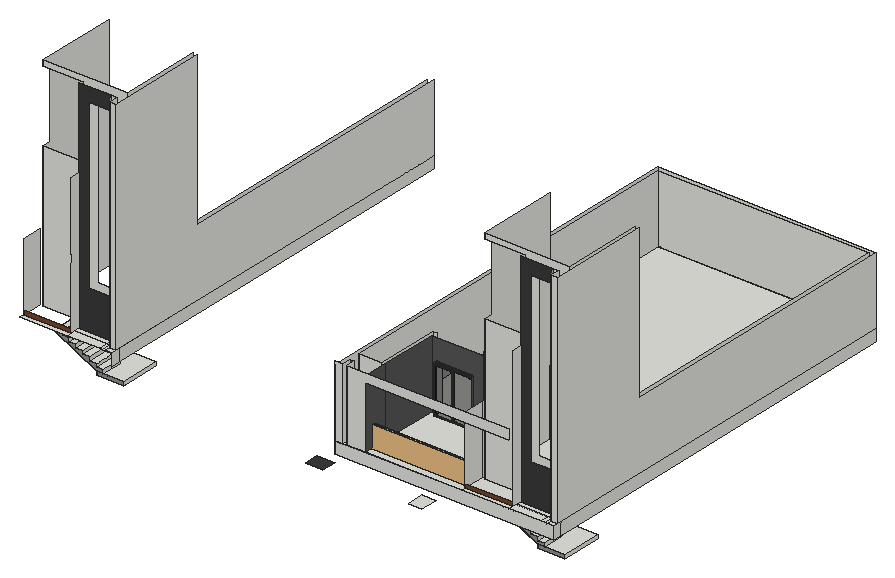
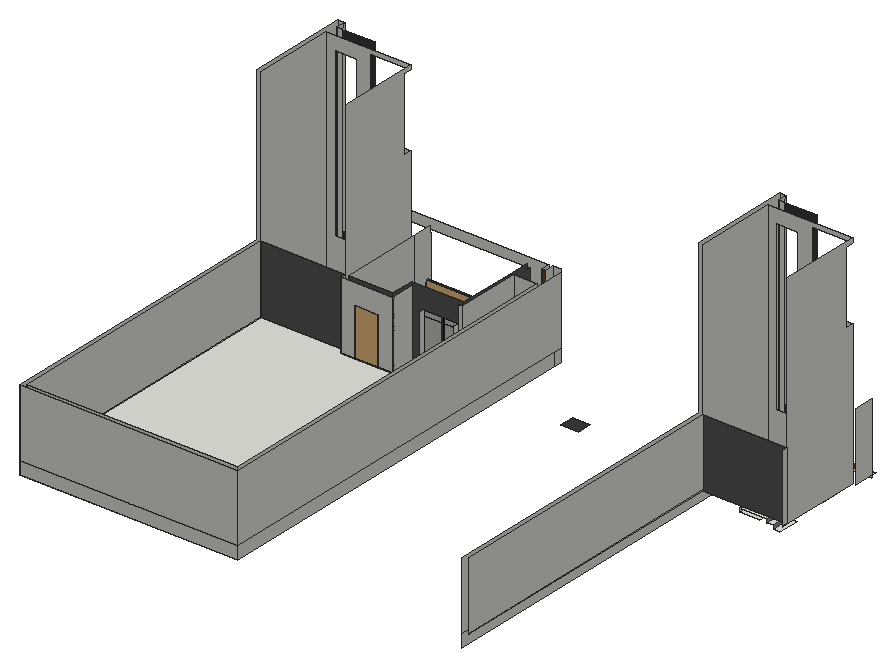
# SketchUp Ruby script. Lengths in inches.
U = 1.inch
M = Sketchup.active_model
def pt(a) = Geom::Point3d.new(a.map { |v| v * U })
def face(e, loops, mat)
  f = e.add_face(loops[0].map { |a| pt(a) })
  loops[1..].each { |l| e.add_face(l.map { |a| pt(a) }).erase! }
  f.material = f.back_material = mat if mat
  f
end
# faces: each face lists its corners as indices into pts; further lists are holes
def faces(e, pts, list, mat = nil) = list.each { |f| face(e, (f[0].is_a?(Array) ? f : [f]).map { |l| l.map { |i| pts[i] } }, mat) }
# xy, xz, yz: faces in a plane at the given z, y or x. An outline is a flat list of corners, or four numbers for a rectangle; further outlines are holes
def ring(l) = l.size == 4 ? [[l[0], l[1]], [l[2], l[1]], [l[2], l[3]], [l[0], l[3]]] : l.each_slice(2).to_a
def flat(e, list, mat, &to3) = list.each { |f| face(e, (f[0].is_a?(Array) ? f : [f]).map { |l| ring(l).map { |u, v| to3.(u, v) } }, mat) }
def xy(e, z, list, mat = nil) = flat(e, list, mat) { |x, y| [x, y, z] }
def xz(e, y, list, mat = nil) = flat(e, list, mat) { |x, z| [x, y, z] }
def yz(e, x, list, mat = nil) = flat(e, list, mat) { |y, z| [x, y, z] }
def lines(e, pts, list) = list.each { |a, b| e.add_line(pt(pts[a]), pt(pts[b])) }
# prism: a flat outline (further loops are holes) pulled along v
def prism(e, loops, v, mat = nil)
  f = face(e, loops, mat); d = Geom::Vector3d.new(v.map { |x| x * U })
  f.pushpull(f.normal.samedirection?(d) ? d.length : -d.length)
end
def box(e, o, s, mat = nil) = prism(e, [[o, [o[0] + s[0], o[1], o[2]], [o[0] + s[0], o[1] + s[1], o[2]], [o[0], o[1] + s[1], o[2]]]], [0, 0, s[2]], mat)
def at(x, y, z, deg = 0) = Geom::Transformation.translation(pt([x, y, z])) * Geom::Transformation.rotation(ORIGIN, Z_AXIS, deg.degrees)
def axes(o, x, y, z) = Geom::Transformation.new([*x, 0, *y, 0, *z, 0, *pt(o).to_a, 1])
def part(name) = M.definitions.add(name)
# library, detail: a bought-in or finely detailed component or shape, given as its bounding box
def library(name, o, s) = part(name).tap { |d| box(d.entities, o, s) }
def detail(e, o, s) = box(e.add_group.entities, o, s)
def put(e, d, t, mat = nil) = e.add_instance(d, t).tap { |i| i.material = mat if mat }
def group(e, t, mat = nil) = e.add_group.tap { |g| g.transformation = t; g.material = mat if mat }.entities
root = M.entities
M.materials.add("Glass_Tinted_Gray").color = [0, 0, 0]
M.materials["Glass_Tinted_Gray"].alpha = 0.125
M.materials.add("[0135_DarkGray]").color = [81, 81, 81]
M.materials.add("[Blacktop Old 02]").color = [143, 145, 145]
M.materials.add("[Color M06]").color = [86, 86, 86]
M.materials.add("[Color M07]").color = [58, 58, 58]
M.materials.add("[Mirror 02]").color = [229, 229, 229]
M.materials.add("[Terrazzo Light Blue]").color = [196, 214, 227]
M.materials.add("[Wood Floor Dark]").color = [153, 94, 42]
M.materials.add("[Wood Veneer 01]").color = [120, 70, 37]
c1 = part("PENTEK_RP Fineline 50S_Sliding_DoorCase_E1")
box(c1.entities,[0,0,0],[1.51,3.66,99.27],"[0135_DarkGray]")
c2 = part("PENTEK_RP Fineline 50S_SlidingDooe_Case_E2")
box(c2.entities,[0,0,0],[96.25,3.66,1.51],"[0135_DarkGray]")
c3 = part("pentek_RP Fineline 50S_SlidingDoor_Case")
put(c3.entities,c1,at(97.76,0,0))
put(c3.entities,c2,at(1.51,0,0))
put(c3.entities,c1,at(0,0,0))
put(c3.entities,c2,at(1.51,0,97.76))
c4 = part("PENTEK_RP Fineline 50S_SlidingDoor_GlazingBead_2")
box(c4.entities,[0,0,0],[0.56,0.59,94.39],"[0135_DarkGray]")
c5 = part("PENTEK_RP Fineline 50S_SlidingDoor_Glass")
box(c5.entities,[0,0,0],[46.58,0.16,94.39],"Glass_Tinted_Gray")
c6 = part("PENTEK_RP Fineline 50S_SlidingDoor_GlazingBead")
box(c6.entities,[0,0,0],[45.47,0.59,0.56],"[0135_DarkGray]")
c7 = part("PENTEK_RP Fineline 50S_SlidingDoor_Leaf_E1")
xy(c7.entities,0,[[0,0,0.93,1.97],[0.93,1.57,1.49,1.97]],"[0135_DarkGray]")
xy(c7.entities,96.25,[[0,0,0.93,0,0.93,1.57,1.49,1.57,1.49,1.97,0,1.97]],"[0135_DarkGray]")
xz(c7.entities,0,[[0,0,0.93,96.25]],"[0135_DarkGray]")
xz(c7.entities,1.57,[[0.93,0,1.49,95.32],[0.93,95.32,1.49,96.25]],"[0135_DarkGray]")
xz(c7.entities,1.97,[[0,0,1.49,96.25]],"[0135_DarkGray]")
yz(c7.entities,0,[[0,0,1.97,96.25]],"[0135_DarkGray]")
yz(c7.entities,0.93,[[0,0,1.57,0.93],[0,0.93,1.57,95.32],[0,95.32,1.57,96.25]],"[0135_DarkGray]")
yz(c7.entities,1.49,[[1.57,0,1.97,95.32],[1.57,95.32,1.97,96.25]],"[0135_DarkGray]")
c8 = part("PENTEK_RP Fineline 50S_SlidingDoor_Leaf_E2")
xy(c8.entities,0,[[0,0,0,1.57,0.56,1.57,0.56,1.97,46.02,1.97,46.02,1.57,46.58,1.57,46.58,0]],"[0135_DarkGray]")
xy(c8.entities,0.93,[[0,0,46.58,1.57]],"[0135_DarkGray]")
xy(c8.entities,1.49,[[0.56,1.57,46.02,1.97]],"[0135_DarkGray]")
xz(c8.entities,0,[[0,0,46.58,0.93]],"[0135_DarkGray]")
xz(c8.entities,1.57,[[0,0,0.56,0.93],[46.02,0,46.58,0.93],[0.56,0.93,46.02,1.49]],"[0135_DarkGray]")
xz(c8.entities,1.97,[[0.56,0,46.02,1.49]],"[0135_DarkGray]")
yz(c8.entities,0,[[0,0,1.57,0.93]],"[0135_DarkGray]")
yz(c8.entities,0.56,[[1.57,0,1.97,0.93],[1.57,0.93,1.97,1.49]],"[0135_DarkGray]")
yz(c8.entities,46.02,[[1.57,0,1.97,0.93],[1.57,0.93,1.97,1.49]],"[0135_DarkGray]")
yz(c8.entities,46.58,[[0,0,1.57,0.93]],"[0135_DarkGray]")
c9 = part("PENTEK_RP Fineline S_SlidingDoor_Leaf1")
put(c9.entities,c4,at(0.93,0,0.93))
put(c9.entities,c4,at(46.96,0,0.93))
put(c9.entities,c5,at(1.49,1.42,0.93))
put(c9.entities,c6,at(1.49,0,0.93))
put(c9.entities,c5,at(1.49,0.59,0.93),"[Terrazzo Light Blue]")
put(c9.entities,c7,at(0,0,0))
put(c9.entities,c7,axes([48.44,0,0],[-1,0,0],[0,1,0],[0,0,1]))
put(c9.entities,c8,axes([0.93,0,96.25],[1,0,0],[0,1,0],[0,0,-1]))
put(c9.entities,c8,at(0.93,0,0))
put(c9.entities,c6,at(1.49,0,94.77))
c10 = part("PENTEK_RP Fineline 50S_SlidingDoor_Leaf2")
put(c10.entities,c5,at(1.49,1.42,0.93))
put(c10.entities,c6,at(1.49,0,94.77))
put(c10.entities,c4,at(46.96,0,0.93))
put(c10.entities,c5,at(1.49,0.59,0.93),"[Mirror 02]")
put(c10.entities,c4,at(0.93,0,0.93))
put(c10.entities,c7,at(0,0,0))
put(c10.entities,c7,axes([48.44,0,0],[-1,0,0],[0,1,0],[0,0,1]))
put(c10.entities,c6,at(1.49,0,0.93))
put(c10.entities,c8,axes([0.93,0,96.25],[1,0,0],[0,1,0],[0,0,-1]))
put(c10.entities,c8,at(0.93,0,0))
c11 = part("PENTEK - Slimmest Steel Sliding Door / Window\#1")
put(c11.entities,c3,at(0,-1.88,-0.09))
put(c11.entities,c9,at(1.51,-2.27,1.42))
put(c11.entities,c10,at(49.32,-0.3,1.42))
c12 = library("Glass Railing",[0,0,0],[139.5,4.76,42])
c13 = library("door (1)",[38.93,25.48,0],[40,9.94,82.68])
xy(root,69.625,[[2545.07,297.1875,2568.82,327.09]])
xy(root,69.625,[[2363.46,297,2394.2,321.97]],"[Color M07]")
xy(root,71.875,[[1967.4,335.33,1979.4,371.33],[2747.78,335.33,2759.78,371.33]])
xy(root,77.875,[[1991.4,299.33,1991.4,335.33,2003.4,335.33,2003.4,371.33,2039.4,371.33,2039.4,299.33],[2771.78,299.33,2771.78,335.33,2783.78,335.33,2783.78,371.33,2819.78,371.33,2819.78,299.33],[1979.4,335.33,1991.4,371.33],[2759.78,335.33,2771.78,371.33]])
xy(root,83.875,[[1991.4,299.33,2003.4,335.33],[2003.4,299.33,2039.4,299.33,2039.4,371.33,1991.4,371.33,1991.4,335.33,2003.4,335.33],[2771.78,299.33,2783.78,335.33],[2783.78,299.33,2819.78,299.33,2819.78,371.33,2771.78,371.33,2771.78,335.33,2783.78,335.33]])
xy(root,89.875,[[1991.4,299.33,2003.4,335.33],[2771.78,299.33,2783.78,335.33]])
xy(root,94.0625,[[2488.8,431.33,2550.55,440.27]])
xy(root,95.875,[[1979.4,299.33,1991.4,335.33],[2759.78,299.33,2771.78,335.33]])
xy(root,101.875,[[1967.4,299.33,1979.4,335.33],[2747.78,299.33,2759.78,335.33]])
xy(root,107.875,[[1955.4,299.33,1967.4,335.33],[2735.78,299.33,2747.78,335.33]])
xy(root,113.875,[[1943.4,299.33,1955.4,335.33],[2723.78,299.33,2735.78,335.33]])
xy(root,119.875,[[1931.4,299.33,1943.4,335.33],[2711.78,299.33,2723.78,335.33]])
xy(root,125.875,[[2441.46,264.125,2827.34,279.8125],[1919.4,299.33,1931.4,335.33],[2699.78,299.33,2711.78,335.33],[[2627.78,371.33,2627.78,431.33,2441.46,431.33,2441.46,975.9375,2827.34,975.9375,2827.34,371.33],[2633.78,379.21,2822.07,379.21,2822.07,970.67,2446.73,970.67,2446.73,440.27,2633.78,440.27]]])
xy(root,125.875,[[[2441.46,279.8125,2441.46,431.33,2627.78,431.33,2627.78,371.33,2827.34,371.33,2827.34,279.8125],[2699.78,299.33,2711.78,335.33],[2446.73,334.62,2454.1,350.3]]],"[Wood Floor Dark]")
xy(root,147.1875,[[2448.71,308.24,2448.71,968.69,2820.09,968.69,2820.09,452.5625,2670.45,452.5625,2670.45,462.67,2579.54,462.67,2579.54,420.39,2538.36,421.04,2488.82,421.04,2488.82,308.24]])
xy(root,147.625,[[1884.4,264.125,1968.34,272.125],[1968.34,264.125,2025.4,279.8125],[2025.4,264.125,2031.45,279.8125],[2031.45,264.125,2035.66,264.125,2035.66,273.0625,2031.45,279.8125],[2035.66,264.125,2046.96,273.0625],
  [2441.46,264.125,2455.02,279.8125],[2455.02,264.125,2462.375,279.8125],[2462.375,264.125,2494.84,279.8125],[2494.84,264.125,2664.78,279.8125],[2664.78,264.125,2748.72,272.125],
  [2748.72,264.125,2805.78,279.8125],[2805.78,264.125,2811.82,279.8125],[2811.82,264.125,2816.04,264.125,2816.04,273.0625,2811.82,279.8125],[2816.04,264.125,2827.34,273.0625],[1884.4,272.125,1968.34,273.0625],
  [2664.78,272.125,2748.72,273.0625],[1884.4,273.0625,1968.34,279.8125],[2035.66,273.0625,2035.66,279.8125,2031.45,279.8125],[2035.66,273.0625,2046.96,279.8125],[2664.78,273.0625,2748.72,279.8125],
  [2816.04,273.0625,2816.04,279.8125,2811.82,279.8125],[2816.04,273.0625,2827.34,279.8125],[1968.34,279.8125,2025.4,289.5],[2025.4,279.8125,2031.45,279.8125,2025.4,289.5],[2031.45,279.8125,2025.4,289.5,2035.66,289.5,2035.66,279.8125],
  [2441.46,279.8125,2441.46,975.9375,2827.34,975.9375,2827.34,279.8125,2816.04,279.8125,2816.04,289.5,2748.72,289.5,2748.72,279.8125,2664.78,279.8125,2664.78,452.5625,2646.47,452.5625,2646.47,462.67,2670.45,462.67,2670.45,308.24,2820.09,308.24,2820.09,968.69,2448.71,968.69,2448.71,308.24,2488.82,308.24,2488.82,421.04,2503.97,421.04,2503.97,411.0625,2494.84,411.0625,2494.84,279.8125],[2494.84,279.8125,2664.78,308.24],[2748.72,279.8125,2805.78,289.5],[2805.78,279.8125,2811.82,279.8125,2805.78,289.5],[2811.82,279.8125,2805.78,289.5,2816.04,289.5,2816.04,279.8125],
  [2448.71,308.24,2448.71,968.69,2820.09,968.69,2820.09,308.24,2670.45,308.24,2670.45,462.67,2579.54,462.67,2579.54,420.39,2565.72,420.61,2538.36,421.04,2488.82,421.04,2488.82,308.24],[2494.84,308.24,2664.78,308.24,2664.78,452.5625,2646.47,452.5625,2646.47,462.67,2604.72,462.67,2604.72,452.5625,2586.59,452.5625,2586.59,411.0625,2565.72,411.0625,2565.72,420.61,2503.97,420.61,2503.97,411.0625,2494.84,411.0625],[2565.72,411.0625,2565.72,420.61,2579.54,420.39,2579.54,462.67,2604.72,462.67,2604.72,452.5625,2586.59,452.5625,2586.59,411.0625],[2503.97,420.61,2503.97,421.04,2538.36,421.04,2565.72,420.61]])
xz(root,264.125,[[2441.46,125.875,2827.34,147.625],[2441.46,147.625,2455.02,273.625],[2462.375,147.625,2494.84,147.625,2494.84,256.875,2748.72,256.875,2748.72,273.625,2462.375,273.625]])
xz(root,272.125,[[1884.4,147.625,1968.34,154.375],[2664.78,147.625,2748.72,154.375]],"[Wood Veneer 01]")
xz(root,273.0625,[[1884.4,143.05,1968.34,147.625],[2664.78,143.05,2748.72,147.625],[2035.66,147.625,2046.96,536.4375],[2816.04,147.625,2827.34,536.4375]])
xz(root,279.8125,[[2441.46,125.875,2827.34,147.625]])
xz(root,279.8125,[[2455.02,147.625,2462.375,273.625]],"[Wood Veneer 01]")
xz(root,289.5,[[2025.4,147.625,2035.66,536.4375],[2805.78,147.625,2816.04,536.4375]])
xz(root,289.5,[[1968.34,147.625,2025.4,147.625,2025.4,217.36,1986.53,217.36,1986.53,512.23,2025.4,512.23,2025.4,536.4375,1968.34,536.4375],[2748.72,147.625,2805.78,147.625,2805.78,217.36,2766.9,217.36,2766.9,512.23,2805.78,512.23,2805.78,536.4375,2748.72,536.4375]],"[Color M07]")
xz(root,299.33,[[1991.4,77.875,2039.4,83.875],[2771.78,77.875,2819.78,83.875],[1991.4,83.875,2003.4,83.875,2003.4,89.875,1991.4,89.875,1991.4,95.875,1979.4,95.875,1979.4,101.875,1967.4,101.875,1967.4,107.875,1955.4,107.875,1955.4,113.875,1943.4,113.875,1943.4,119.875,1931.4,119.875,1931.4,125.875,1919.4,125.875,1919.4,119.875],[2771.78,83.875,2783.78,83.875,2783.78,89.875,2771.78,89.875,2771.78,95.875,2759.78,95.875,2759.78,101.875,2747.78,101.875,2747.78,107.875,2735.78,107.875,2735.78,113.875,2723.78,113.875,2723.78,119.875,2711.78,119.875,2711.78,125.875,2699.78,125.875,2699.78,119.875]],"[Blacktop Old 02]")
xz(root,308.24,[[2448.71,147.1875,2488.82,147.625],[[1890.08,147.625,1890.08,400.68,1962.22,400.68,1962.22,528.11,1890.08,528.11,1890.08,536.4375,2039.72,536.4375,2039.72,147.625],[1986.53,217.36,2025.4,512.23]],[2448.71,147.625,2488.82,267.625],[[2670.45,147.625,2670.45,400.68,2742.59,400.68,2742.59,528.11,2670.45,528.11,2670.45,536.4375,2820.09,536.4375,2820.09,147.625],[2766.9,217.36,2805.78,512.23]]])
xz(root,335.33,[[1991.4,83.875,1919.4,119.875,1919.4,125.875,1931.4,125.875,1931.4,119.875,1943.4,119.875,1943.4,113.875,1955.4,113.875,1955.4,107.875,1967.4,107.875,1967.4,101.875,1979.4,101.875,1979.4,95.875,1991.4,95.875,1991.4,89.875,2003.4,89.875,2003.4,83.875],[2771.78,83.875,2699.78,119.875,2699.78,125.875,2711.78,125.875,2711.78,119.875,2723.78,119.875,2723.78,113.875,2735.78,113.875,2735.78,107.875,2747.78,107.875,2747.78,101.875,2759.78,101.875,2759.78,95.875,2771.78,95.875,2771.78,89.875,2783.78,89.875,2783.78,83.875]])
xz(root,411.0625,[[2494.84,147.625,2503.97,147.625,2503.97,230.5625,2565.72,230.5625,2565.72,147.625,2586.59,147.625,2586.59,267.625,2494.84,267.625]],"[Color M06]")
xz(root,421.04,[[2488.82,147.1875,2496.09,147.625],[2496.09,147.1875,2538.36,147.625],[2488.82,147.625,2496.09,267.625]])
xz(root,452.5625,[[1890.08,147.1875,2039.72,267.625],[2670.45,147.1875,2820.09,267.625],[2586.59,147.625,2604.72,147.625,2604.72,231.75,2646.47,231.75,2646.47,147.625,2664.78,147.625,2664.78,267.625,2586.59,267.625]],"[Color M06]")
xz(root,462.67,[[2579.54,147.1875,2670.45,147.625],[2579.54,147.625,2604.72,147.625,2604.72,231.75,2646.47,231.75,2646.47,147.625,2670.45,147.625,2670.45,267.625,2579.54,267.625]])
xz(root,968.69,[[2448.71,147.1875,2820.09,147.625],[2448.71,147.625,2820.09,267.625]])
xz(root,975.9375,[[2441.46,125.875,2827.34,147.625],[2441.46,147.625,2827.34,267.625]])
yz(root,1884.4,[[272.125,147.625,272.125,154.375,273.0625,154.375,273.0625,155.86,272.125,155.86,272.125,167.1875,273.0625,167.1875,273.0625,168.67,272.125,168.67,272.125,180,273.0625,180,273.0625,181.48,272.125,181.48,272.125,192.8125,273.0625,192.8125,273.0625,194.3,272.125,194.3,272.125,205.625,273.0625,205.625,273.0625,207.11,272.125,207.11,272.125,218.4375,273.0625,218.4375,273.0625,219.92,272.125,219.92,272.125,231.25,273.0625,231.25,273.0625,232.73,272.125,232.73,272.125,244.0625,273.0625,244.0625,273.0625,245.55,272.125,245.55,272.125,256.875,273.0625,256.875,273.0625,267.625,308.24,267.625,308.24,147.625]])
yz(root,1890.08,[[452.5625,147.1875,462.67,147.625],[308.24,147.625,452.5625,147.625,452.5625,536.4375,308.24,536.4375,308.24,528.11,323.81,528.11,323.81,400.68,308.24,400.68],[452.5625,147.625,462.67,267.625]])
yz(root,1919.4,[[299.33,119.875,335.33,125.875]])
yz(root,1931.4,[[299.33,119.875,335.33,125.875]])
yz(root,1943.4,[[299.33,113.875,335.33,119.875]])
yz(root,1955.4,[[299.33,107.875,335.33,113.875]])
yz(root,1967.4,[[299.33,101.875,335.33,107.875]])
yz(root,1968.34,[[272.125,147.625,289.5,147.625,289.5,393.625,271.6875,393.625,271.6875,273.625,273.0625,273.625,273.0625,256.875,272.125,256.875,272.125,245.55,273.0625,245.55,273.0625,244.0625,272.125,244.0625,272.125,232.73,273.0625,232.73,273.0625,231.25,272.125,231.25,272.125,219.92,273.0625,219.92,273.0625,218.4375,272.125,218.4375,272.125,207.11,273.0625,207.11,273.0625,205.625,272.125,205.625,272.125,194.3,273.0625,194.3,273.0625,192.8125,272.125,192.8125,272.125,181.48,273.0625,181.48,273.0625,180,272.125,180,272.125,168.67,273.0625,168.67,273.0625,167.1875,272.125,167.1875,272.125,155.86,273.0625,155.86,273.0625,154.375,272.125,154.375]])
yz(root,1979.4,[[299.33,95.875,335.33,101.875]])
yz(root,1979.4,[[335.33,71.875,371.33,77.875]],"[Blacktop Old 02]")
yz(root,1991.4,[[299.33,89.875,335.33,95.875]])
yz(root,1991.4,[[299.33,77.875,335.33,83.875],[335.33,77.875,371.33,83.875]],"[Blacktop Old 02]")
yz(root,2003.4,[[299.33,83.875,335.33,89.875]])
yz(root,2035.66,[[273.0625,147.625,289.5,536.4375]])
yz(root,2039.4,[[299.33,77.875,371.33,83.875]])
yz(root,2039.72,[[452.5625,147.1875,968.69,147.625],[308.24,147.625,452.5625,536.4375],[452.5625,147.625,968.69,267.625]])
yz(root,2046.96,[[264.125,125.875,279.8125,147.625],[279.8125,125.875,975.9375,147.625],[273.0625,147.625,975.9375,147.625,975.9375,267.625,452.5625,267.625,452.5625,536.4375,273.0625,536.4375]])
yz(root,2441.46,[[264.125,125.875,279.8125,147.625],[279.8125,125.875,975.9375,147.625],[264.125,147.625,975.9375,267.625]])
yz(root,2448.71,[[308.24,147.1875,968.69,147.625],[308.24,147.625,968.69,267.625]])
yz(root,2455.02,[[264.125,147.625,279.8125,273.625]])
yz(root,2462.375,[[264.125,147.625,279.8125,273.625]])
yz(root,2488.82,[[308.24,147.1875,421.04,147.625],[308.24,147.625,421.04,267.625]])
yz(root,2494.84,[[264.125,147.625,308.24,147.625,308.24,267.625,272.68,267.625,272.68,256.875,264.125,256.875],[308.24,147.625,411.0625,267.625]],"[Color M06]")
yz(root,2503.97,[[411.0625,147.625,420.61,230.5625]])
yz(root,2565.72,[[411.0625,147.625,420.61,230.5625]])
yz(root,2579.54,[[420.39,147.1875,459.32,147.625],[459.32,147.1875,462.67,147.625],[420.39,147.625,459.32,267.625],[459.32,147.625,462.67,267.625]])
yz(root,2586.59,[[411.0625,147.625,452.5625,267.625]],"[Color M06]")
yz(root,2604.72,[[452.5625,147.625,462.67,231.75]])
yz(root,2646.47,[[452.5625,147.625,462.67,231.75]])
yz(root,2664.78,[[272.125,147.625,272.125,154.375,273.0625,154.375,273.0625,155.86,272.125,155.86,272.125,167.1875,273.0625,167.1875,273.0625,168.67,272.125,168.67,272.125,180,273.0625,180,273.0625,181.48,272.125,181.48,272.125,192.8125,273.0625,192.8125,273.0625,194.3,272.125,194.3,272.125,205.625,273.0625,205.625,273.0625,207.11,272.125,207.11,272.125,218.4375,273.0625,218.4375,273.0625,219.92,272.125,219.92,272.125,231.25,273.0625,231.25,273.0625,232.73,272.125,232.73,272.125,244.0625,273.0625,244.0625,273.0625,245.55,272.125,245.55,272.125,256.875,273.0625,256.875,273.0625,267.625,308.24,267.625,308.24,147.625],[308.24,147.625,452.5625,267.625]])
yz(root,2670.45,[[452.5625,147.1875,462.67,147.625],[308.24,147.625,452.5625,147.625,452.5625,536.4375,308.24,536.4375,308.24,528.11,323.81,528.11,323.81,400.68,308.24,400.68],[452.5625,147.625,462.67,267.625]])
yz(root,2699.78,[[299.33,119.875,335.33,125.875]])
yz(root,2711.78,[[299.33,119.875,335.33,125.875]])
yz(root,2723.78,[[299.33,113.875,335.33,119.875]])
yz(root,2735.78,[[299.33,107.875,335.33,113.875]])
yz(root,2747.78,[[299.33,101.875,335.33,107.875]])
yz(root,2748.72,[[272.125,147.625,289.5,147.625,289.5,393.625,271.6875,393.625,271.6875,273.625,273.0625,273.625,273.0625,256.875,272.125,256.875,272.125,245.55,273.0625,245.55,273.0625,244.0625,272.125,244.0625,272.125,232.73,273.0625,232.73,273.0625,231.25,272.125,231.25,272.125,219.92,273.0625,219.92,273.0625,218.4375,272.125,218.4375,272.125,207.11,273.0625,207.11,273.0625,205.625,272.125,205.625,272.125,194.3,273.0625,194.3,273.0625,192.8125,272.125,192.8125,272.125,181.48,273.0625,181.48,273.0625,180,272.125,180,272.125,168.67,273.0625,168.67,273.0625,167.1875,272.125,167.1875,272.125,155.86,273.0625,155.86,273.0625,154.375,272.125,154.375]])
yz(root,2759.78,[[299.33,95.875,335.33,101.875]])
yz(root,2759.78,[[335.33,71.875,371.33,77.875]],"[Blacktop Old 02]")
yz(root,2771.78,[[299.33,89.875,335.33,95.875]])
yz(root,2771.78,[[299.33,77.875,335.33,83.875],[335.33,77.875,371.33,83.875]],"[Blacktop Old 02]")
yz(root,2783.78,[[299.33,83.875,335.33,89.875]])
yz(root,2816.04,[[273.0625,147.625,289.5,536.4375]])
yz(root,2819.78,[[299.33,77.875,371.33,83.875]])
yz(root,2820.09,[[452.5625,147.1875,968.69,147.625],[308.24,147.625,452.5625,536.4375],[452.5625,147.625,968.69,267.625]])
yz(root,2827.34,[[264.125,125.875,279.8125,147.625],[279.8125,125.875,975.9375,147.625],[273.0625,147.625,975.9375,147.625,975.9375,267.625,452.5625,267.625,452.5625,536.4375,273.0625,536.4375]])
p = [[1919.4,335.33,119.875],[1991.4,335.33,83.875],[1991.4,299.33,83.875],[1919.4,299.33,119.875],[2699.78,335.33,119.875],[2771.78,335.33,83.875],
  [2771.78,299.33,83.875],[2699.78,299.33,119.875],[2579.54,420.39,147.1875],[2579.54,420.39,147.625],[2565.72,420.61,147.625],[2538.36,421.04,147.625],
  [2538.36,421.04,147.1875],[2035.66,273.0625,536.4375],[2025.4,289.5,536.4375],[2025.4,289.5,512.23],[2025.4,289.5,217.36],[2025.4,289.5,147.625],
  [2031.45,279.8125,147.625],[2035.66,273.0625,147.625],[2816.04,273.0625,536.4375],[2805.78,289.5,536.4375],[2805.78,289.5,512.23],[2805.78,289.5,217.36],
  [2805.78,289.5,147.625],[2811.82,279.8125,147.625],[2816.04,273.0625,147.625],[1919.4,335.33,131.875],[1907.4,335.33,131.875],[1919.4,335.33,125.875],
  [2699.78,335.33,125.875],[2699.78,335.33,131.875],[2687.78,335.33,131.875]]
faces(root,p,[[0,1,2,3],[4,5,6,7]],"[Blacktop Old 02]")
faces(root,p,[[8,9,10,11,12],[13,14,15,16,17,18,19],[20,21,22,23,24,25,26]])
lines(root,p,[[27,28],[29,27],[30,31],[31,32]])
put(root,c11,axes([2503.02,405.56,146.3],[0.6868,0,0],[0,0.6868,0],[0,0,0.85163]))
put(root,c12,axes([2494.27,277.75,143.83],[1.22225,0,0],[0,1,0],[0,0,1]))
put(root,c13,axes([2564.09,427.08,147.625],[1.04375,0,0],[0,1,0],[0,0,1.01751]))
